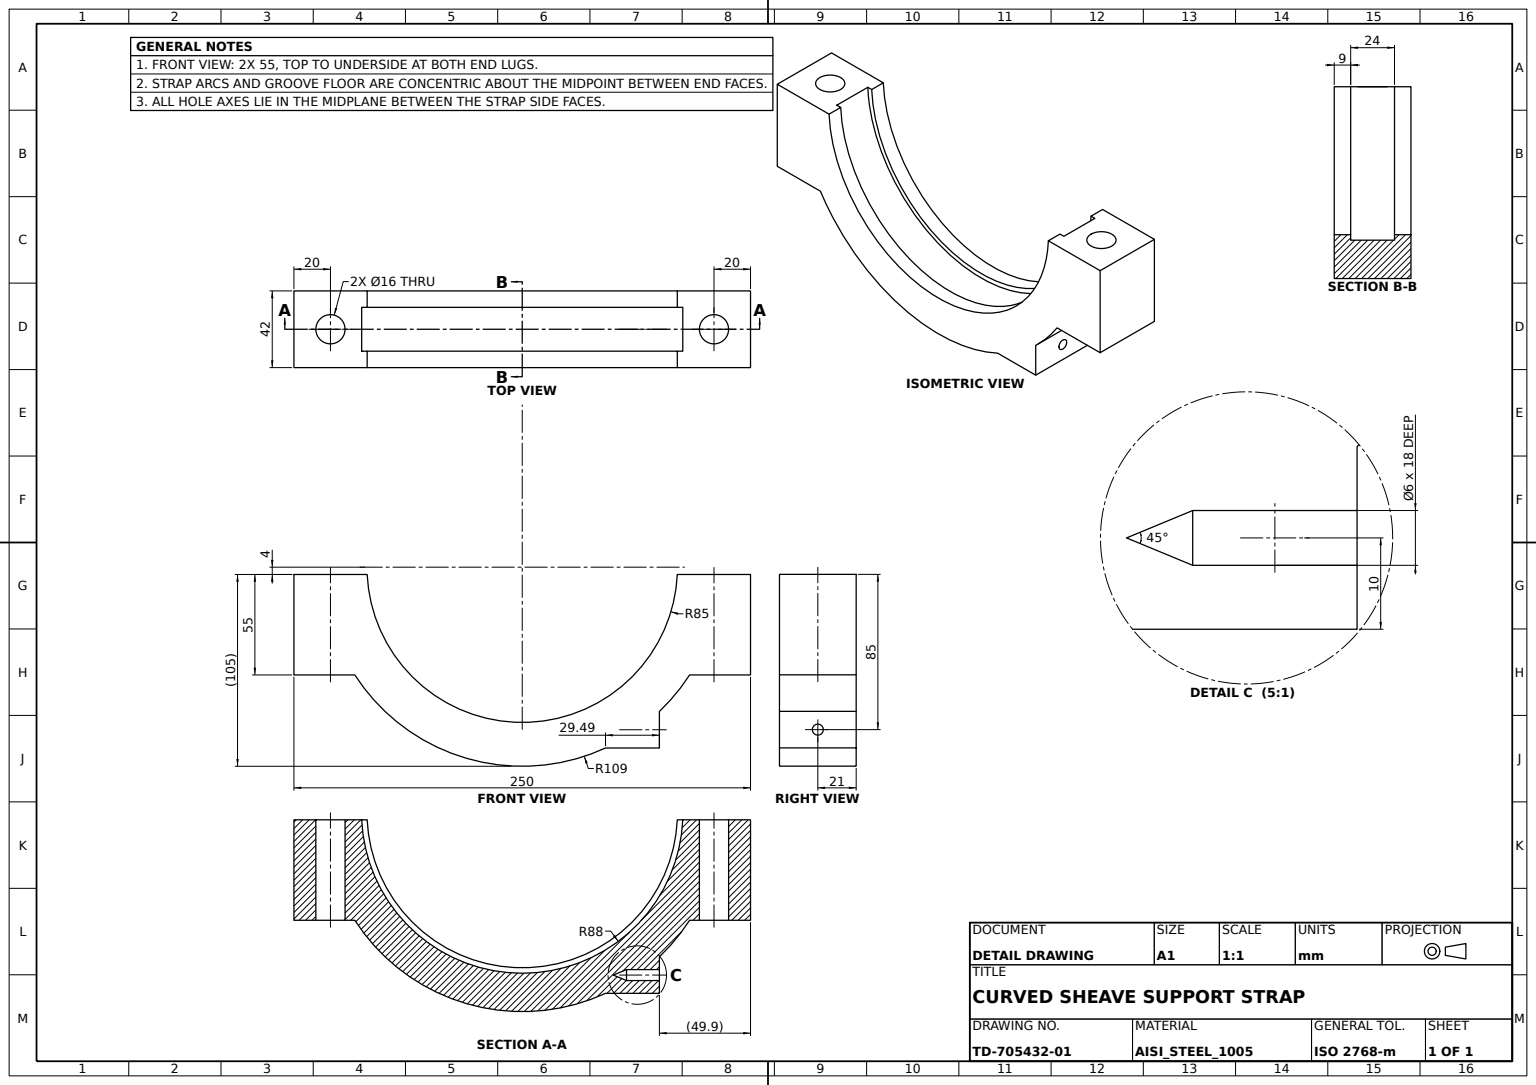
ISO-10303-21;
HEADER;
FILE_DESCRIPTION((''),'2;1');
FILE_NAME('','',(''),(''),'','','');
FILE_SCHEMA(('AUTOMOTIVE_DESIGN'));
ENDSEC;
DATA;
#1=APPLICATION_CONTEXT('');
#2=PRODUCT_CONTEXT('',#1,'mechanical');
#3=PRODUCT('','','',(#2));
#4=PRODUCT_DEFINITION_FORMATION('','',#3);
#5=PRODUCT_DEFINITION_CONTEXT('',#1,'design');
#6=PRODUCT_DEFINITION('','',#4,#5);
#7=PRODUCT_DEFINITION_SHAPE('','',#6);
#8=(LENGTH_UNIT()NAMED_UNIT(*)SI_UNIT(.MILLI.,.METRE.));
#9=(NAMED_UNIT(*)PLANE_ANGLE_UNIT()SI_UNIT($,.RADIAN.));
#10=(NAMED_UNIT(*)SI_UNIT($,.STERADIAN.)SOLID_ANGLE_UNIT());
#11=UNCERTAINTY_MEASURE_WITH_UNIT(LENGTH_MEASURE(0.005),#8,'distance_accuracy_value','');
#12=(GEOMETRIC_REPRESENTATION_CONTEXT(3)GLOBAL_UNCERTAINTY_ASSIGNED_CONTEXT((#11))GLOBAL_UNIT_ASSIGNED_CONTEXT((#8,#9,#10))REPRESENTATION_CONTEXT('',''));
#13=CARTESIAN_POINT('',(-55.,91.651514,21.));
#14=VERTEX_POINT('',#13);
#15=CARTESIAN_POINT('',(-55.,91.651514,-21.));
#16=VERTEX_POINT('',#15);
#17=DIRECTION('',(0.,0.,-1.));
#18=VECTOR('',#17,1000.);
#19=LINE('',#13,#18);
#20=EDGE_CURVE('',#14,#16,#19,.T.);
#21=ORIENTED_EDGE('',*,*,#20,.T.);
#22=CARTESIAN_POINT('',(-75.,75.099933,-21.));
#23=VERTEX_POINT('',#22);
#24=CARTESIAN_POINT('',(4.,0.,-21.));
#25=DIRECTION('',(0.,0.,1.));
#26=DIRECTION('',(0.,1.,0.));
#27=AXIS2_PLACEMENT_3D('',#24,#25,#26);
#28=CIRCLE('',#27,109.);
#29=EDGE_CURVE('',#16,#23,#28,.T.);
#30=ORIENTED_EDGE('',*,*,#29,.T.);
#31=CARTESIAN_POINT('',(-75.,75.099933,21.));
#32=VERTEX_POINT('',#31);
#33=LINE('',#31,#18);
#34=EDGE_CURVE('',#32,#23,#33,.T.);
#35=ORIENTED_EDGE('',*,*,#34,.F.);
#36=CARTESIAN_POINT('',(4.,0.,21.));
#37=AXIS2_PLACEMENT_3D('',#36,#25,#26);
#38=CIRCLE('',#37,109.);
#39=EDGE_CURVE('',#14,#32,#38,.T.);
#40=ORIENTED_EDGE('',*,*,#39,.F.);
#41=EDGE_LOOP('',(#21,#30,#35,#40));
#42=FACE_BOUND('',#41,.T.);
#43=DIRECTION('',(-1.,0.,0.));
#44=AXIS2_PLACEMENT_3D('',#36,#17,#43);
#45=CYLINDRICAL_SURFACE('',#44,109.);
#46=ADVANCED_FACE('',(#42),#45,.T.);
#47=CARTESIAN_POINT('',(0.,87.909044,12.));
#48=VERTEX_POINT('',#47);
#49=CARTESIAN_POINT('',(0.,87.909044,-12.));
#50=VERTEX_POINT('',#49);
#51=LINE('',#47,#18);
#52=EDGE_CURVE('',#48,#50,#51,.T.);
#53=ORIENTED_EDGE('',*,*,#52,.F.);
#54=CARTESIAN_POINT('',(0.,-87.909044,12.));
#55=VERTEX_POINT('',#54);
#56=CARTESIAN_POINT('',(4.,0.,12.));
#57=AXIS2_PLACEMENT_3D('',#56,#25,#26);
#58=CIRCLE('',#57,88.);
#59=EDGE_CURVE('',#55,#48,#58,.F.);
#60=ORIENTED_EDGE('',*,*,#59,.F.);
#61=CARTESIAN_POINT('',(0.,-87.909044,-12.));
#62=VERTEX_POINT('',#61);
#63=LINE('',#54,#18);
#64=EDGE_CURVE('',#55,#62,#63,.T.);
#65=ORIENTED_EDGE('',*,*,#64,.T.);
#66=CARTESIAN_POINT('',(4.,0.,-12.));
#67=AXIS2_PLACEMENT_3D('',#66,#25,#26);
#68=CIRCLE('',#67,88.);
#69=EDGE_CURVE('',#62,#50,#68,.F.);
#70=ORIENTED_EDGE('',*,*,#69,.T.);
#71=EDGE_LOOP('',(#53,#60,#65,#70));
#72=FACE_BOUND('',#71,.T.);
#73=AXIS2_PLACEMENT_3D('',#56,#17,#43);
#74=CYLINDRICAL_SURFACE('',#73,88.);
#75=ADVANCED_FACE('',(#72),#74,.F.);
#76=CARTESIAN_POINT('',(0.,-84.90583,-21.));
#77=VERTEX_POINT('',#76);
#78=CARTESIAN_POINT('',(0.,84.90583,-21.));
#79=VERTEX_POINT('',#78);
#80=AXIS2_PLACEMENT_3D('',#24,#17,#26);
#81=CIRCLE('',#80,85.);
#82=EDGE_CURVE('',#77,#79,#81,.T.);
#83=ORIENTED_EDGE('',*,*,#82,.T.);
#84=CARTESIAN_POINT('',(0.,84.90583,-12.));
#85=VERTEX_POINT('',#84);
#86=CARTESIAN_POINT('',(0.,84.90583,21.));
#87=LINE('',#86,#18);
#88=EDGE_CURVE('',#85,#79,#87,.T.);
#89=ORIENTED_EDGE('',*,*,#88,.F.);
#90=CARTESIAN_POINT('',(0.,-84.90583,-12.));
#91=VERTEX_POINT('',#90);
#92=AXIS2_PLACEMENT_3D('',#66,#17,#26);
#93=CIRCLE('',#92,85.);
#94=EDGE_CURVE('',#91,#85,#93,.T.);
#95=ORIENTED_EDGE('',*,*,#94,.F.);
#96=CARTESIAN_POINT('',(0.,-84.90583,21.));
#97=LINE('',#96,#18);
#98=EDGE_CURVE('',#91,#77,#97,.T.);
#99=ORIENTED_EDGE('',*,*,#98,.T.);
#100=EDGE_LOOP('',(#83,#89,#95,#99));
#101=FACE_BOUND('',#100,.T.);
#102=CYLINDRICAL_SURFACE('',#44,85.);
#103=ADVANCED_FACE('',(#101),#102,.F.);
#104=CARTESIAN_POINT('',(-55.,-97.,0.));
#105=VERTEX_POINT('',#104);
#106=CARTESIAN_POINT('',(-55.,-105.,0.));
#107=AXIS2_PLACEMENT_3D('',#106,#43,#26);
#108=CIRCLE('',#107,8.);
#109=EDGE_CURVE('',#105,#105,#108,.T.);
#110=ORIENTED_EDGE('',*,*,#109,.F.);
#111=EDGE_LOOP('',(#110));
#112=FACE_BOUND('',#111,.T.);
#113=CARTESIAN_POINT('',(-55.,-91.651514,21.));
#114=VERTEX_POINT('',#113);
#115=CARTESIAN_POINT('',(-55.,-125.,21.));
#116=VERTEX_POINT('',#115);
#117=DIRECTION('',(0.,-1.,0.));
#118=VECTOR('',#117,1000.);
#119=LINE('',#113,#118);
#120=EDGE_CURVE('',#114,#116,#119,.T.);
#121=ORIENTED_EDGE('',*,*,#120,.F.);
#122=CARTESIAN_POINT('',(-55.,-91.651514,-21.));
#123=VERTEX_POINT('',#122);
#124=LINE('',#113,#18);
#125=EDGE_CURVE('',#114,#123,#124,.T.);
#126=ORIENTED_EDGE('',*,*,#125,.T.);
#127=CARTESIAN_POINT('',(-55.,-125.,-21.));
#128=VERTEX_POINT('',#127);
#129=LINE('',#122,#118);
#130=EDGE_CURVE('',#123,#128,#129,.T.);
#131=ORIENTED_EDGE('',*,*,#130,.T.);
#132=LINE('',#115,#18);
#133=EDGE_CURVE('',#116,#128,#132,.T.);
#134=ORIENTED_EDGE('',*,*,#133,.F.);
#135=EDGE_LOOP('',(#121,#126,#131,#134));
#136=FACE_BOUND('',#135,.T.);
#137=DIRECTION('',(1.,0.,0.));
#138=AXIS2_PLACEMENT_3D('',#113,#137,#17);
#139=PLANE('',#138);
#140=ADVANCED_FACE('',(#112,#136),#139,.F.);
#141=CARTESIAN_POINT('',(0.,97.,0.));
#142=VERTEX_POINT('',#141);
#143=CARTESIAN_POINT('',(0.,105.,0.));
#144=AXIS2_PLACEMENT_3D('',#143,#43,#117);
#145=CIRCLE('',#144,8.);
#146=EDGE_CURVE('',#142,#142,#145,.T.);
#147=ORIENTED_EDGE('',*,*,#146,.F.);
#148=EDGE_LOOP('',(#147));
#149=FACE_BOUND('',#148,.T.);
#150=CARTESIAN_POINT('',(-55.,97.,0.));
#151=VERTEX_POINT('',#150);
#152=CARTESIAN_POINT('',(-55.,105.,0.));
#153=AXIS2_PLACEMENT_3D('',#152,#137,#117);
#154=CIRCLE('',#153,8.);
#155=EDGE_CURVE('',#151,#151,#154,.T.);
#156=ORIENTED_EDGE('',*,*,#155,.F.);
#157=EDGE_LOOP('',(#156));
#158=FACE_BOUND('',#157,.T.);
#159=CARTESIAN_POINT('',(5.5,105.,0.));
#160=AXIS2_PLACEMENT_3D('',#159,#43,#25);
#161=CYLINDRICAL_SURFACE('',#160,8.);
#162=ADVANCED_FACE('',(#149,#158),#161,.F.);
#163=CARTESIAN_POINT('',(-95.,45.607017,-21.));
#164=VERTEX_POINT('',#163);
#165=EDGE_CURVE('',#164,#123,#28,.T.);
#166=ORIENTED_EDGE('',*,*,#165,.T.);
#167=ORIENTED_EDGE('',*,*,#125,.F.);
#168=CARTESIAN_POINT('',(-95.,45.607017,21.));
#169=VERTEX_POINT('',#168);
#170=EDGE_CURVE('',#169,#114,#38,.T.);
#171=ORIENTED_EDGE('',*,*,#170,.F.);
#172=LINE('',#168,#18);
#173=EDGE_CURVE('',#169,#164,#172,.T.);
#174=ORIENTED_EDGE('',*,*,#173,.T.);
#175=EDGE_LOOP('',(#166,#167,#171,#174));
#176=FACE_BOUND('',#175,.T.);
#177=ADVANCED_FACE('',(#176),#45,.T.);
#178=ORIENTED_EDGE('',*,*,#130,.F.);
#179=ORIENTED_EDGE('',*,*,#165,.F.);
#180=CARTESIAN_POINT('',(-95.,75.099933,-21.));
#181=VERTEX_POINT('',#180);
#182=LINE('',#180,#118);
#183=EDGE_CURVE('',#181,#164,#182,.T.);
#184=ORIENTED_EDGE('',*,*,#183,.F.);
#185=VECTOR('',#43,1000.);
#186=LINE('',#22,#185);
#187=EDGE_CURVE('',#23,#181,#186,.T.);
#188=ORIENTED_EDGE('',*,*,#187,.F.);
#189=ORIENTED_EDGE('',*,*,#29,.F.);
#190=CARTESIAN_POINT('',(-55.,125.,-21.));
#191=VERTEX_POINT('',#190);
#192=LINE('',#190,#118);
#193=EDGE_CURVE('',#191,#16,#192,.T.);
#194=ORIENTED_EDGE('',*,*,#193,.F.);
#195=CARTESIAN_POINT('',(0.,125.,-21.));
#196=VERTEX_POINT('',#195);
#197=LINE('',#195,#185);
#198=EDGE_CURVE('',#196,#191,#197,.T.);
#199=ORIENTED_EDGE('',*,*,#198,.F.);
#200=VECTOR('',#26,1000.);
#201=LINE('',#78,#200);
#202=EDGE_CURVE('',#79,#196,#201,.T.);
#203=ORIENTED_EDGE('',*,*,#202,.F.);
#204=ORIENTED_EDGE('',*,*,#82,.F.);
#205=CARTESIAN_POINT('',(0.,-125.,-21.));
#206=VERTEX_POINT('',#205);
#207=LINE('',#205,#200);
#208=EDGE_CURVE('',#206,#77,#207,.T.);
#209=ORIENTED_EDGE('',*,*,#208,.F.);
#210=VECTOR('',#137,1000.);
#211=LINE('',#127,#210);
#212=EDGE_CURVE('',#128,#206,#211,.T.);
#213=ORIENTED_EDGE('',*,*,#212,.F.);
#214=EDGE_LOOP('',(#178,#179,#184,#188,#189,#194,#199,#203,#204,#209,#213));
#215=FACE_BOUND('',#214,.T.);
#216=AXIS2_PLACEMENT_3D('',#24,#25,#137);
#217=PLANE('',#216);
#218=ADVANCED_FACE('',(#215),#217,.F.);
#219=CARTESIAN_POINT('',(-95.,75.099933,21.));
#220=VERTEX_POINT('',#219);
#221=LINE('',#219,#118);
#222=EDGE_CURVE('',#220,#169,#221,.T.);
#223=ORIENTED_EDGE('',*,*,#222,.T.);
#224=ORIENTED_EDGE('',*,*,#170,.T.);
#225=ORIENTED_EDGE('',*,*,#120,.T.);
#226=CARTESIAN_POINT('',(0.,-125.,21.));
#227=VERTEX_POINT('',#226);
#228=LINE('',#115,#210);
#229=EDGE_CURVE('',#116,#227,#228,.T.);
#230=ORIENTED_EDGE('',*,*,#229,.T.);
#231=VERTEX_POINT('',#96);
#232=LINE('',#226,#200);
#233=EDGE_CURVE('',#227,#231,#232,.T.);
#234=ORIENTED_EDGE('',*,*,#233,.T.);
#235=VERTEX_POINT('',#86);
#236=AXIS2_PLACEMENT_3D('',#36,#17,#26);
#237=CIRCLE('',#236,85.);
#238=EDGE_CURVE('',#231,#235,#237,.T.);
#239=ORIENTED_EDGE('',*,*,#238,.T.);
#240=CARTESIAN_POINT('',(0.,125.,21.));
#241=VERTEX_POINT('',#240);
#242=LINE('',#86,#200);
#243=EDGE_CURVE('',#235,#241,#242,.T.);
#244=ORIENTED_EDGE('',*,*,#243,.T.);
#245=CARTESIAN_POINT('',(-55.,125.,21.));
#246=VERTEX_POINT('',#245);
#247=LINE('',#240,#185);
#248=EDGE_CURVE('',#241,#246,#247,.T.);
#249=ORIENTED_EDGE('',*,*,#248,.T.);
#250=LINE('',#245,#118);
#251=EDGE_CURVE('',#246,#14,#250,.T.);
#252=ORIENTED_EDGE('',*,*,#251,.T.);
#253=ORIENTED_EDGE('',*,*,#39,.T.);
#254=LINE('',#31,#185);
#255=EDGE_CURVE('',#32,#220,#254,.T.);
#256=ORIENTED_EDGE('',*,*,#255,.T.);
#257=EDGE_LOOP('',(#223,#224,#225,#230,#234,#239,#244,#249,#252,#253,#256));
#258=FACE_BOUND('',#257,.T.);
#259=AXIS2_PLACEMENT_3D('',#36,#25,#137);
#260=PLANE('',#259);
#261=ADVANCED_FACE('',(#258),#260,.T.);
#262=CARTESIAN_POINT('',(0.,-84.90583,12.));
#263=VERTEX_POINT('',#262);
#264=CARTESIAN_POINT('',(0.,84.90583,12.));
#265=VERTEX_POINT('',#264);
#266=AXIS2_PLACEMENT_3D('',#56,#17,#26);
#267=CIRCLE('',#266,85.);
#268=EDGE_CURVE('',#263,#265,#267,.T.);
#269=ORIENTED_EDGE('',*,*,#268,.F.);
#270=LINE('',#54,#200);
#271=EDGE_CURVE('',#55,#263,#270,.T.);
#272=ORIENTED_EDGE('',*,*,#271,.F.);
#273=ORIENTED_EDGE('',*,*,#59,.T.);
#274=LINE('',#264,#200);
#275=EDGE_CURVE('',#265,#48,#274,.T.);
#276=ORIENTED_EDGE('',*,*,#275,.F.);
#277=EDGE_LOOP('',(#269,#272,#273,#276));
#278=FACE_BOUND('',#277,.T.);
#279=PLANE('',#73);
#280=ADVANCED_FACE('',(#278),#279,.T.);
#281=CARTESIAN_POINT('',(-85.,75.099933,-3.));
#282=VERTEX_POINT('',#281);
#283=CARTESIAN_POINT('',(-85.,75.099933,0.));
#284=AXIS2_PLACEMENT_3D('',#283,#117,#17);
#285=CIRCLE('',#284,3.);
#286=EDGE_CURVE('',#282,#282,#285,.T.);
#287=ORIENTED_EDGE('',*,*,#286,.T.);
#288=EDGE_LOOP('',(#287));
#289=FACE_BOUND('',#288,.T.);
#290=LINE('',#219,#18);
#291=EDGE_CURVE('',#220,#181,#290,.T.);
#292=ORIENTED_EDGE('',*,*,#291,.F.);
#293=ORIENTED_EDGE('',*,*,#255,.F.);
#294=ORIENTED_EDGE('',*,*,#34,.T.);
#295=ORIENTED_EDGE('',*,*,#187,.T.);
#296=EDGE_LOOP('',(#292,#293,#294,#295));
#297=FACE_BOUND('',#296,.T.);
#298=AXIS2_PLACEMENT_3D('',#31,#117,#17);
#299=PLANE('',#298);
#300=ADVANCED_FACE('',(#289,#297),#299,.F.);
#301=ORIENTED_EDGE('',*,*,#109,.T.);
#302=EDGE_LOOP('',(#301));
#303=FACE_BOUND('',#302,.T.);
#304=CARTESIAN_POINT('',(0.,-105.,8.));
#305=VERTEX_POINT('',#304);
#306=CARTESIAN_POINT('',(0.,-105.,0.));
#307=AXIS2_PLACEMENT_3D('',#306,#43,#25);
#308=CIRCLE('',#307,8.);
#309=EDGE_CURVE('',#305,#305,#308,.F.);
#310=ORIENTED_EDGE('',*,*,#309,.T.);
#311=EDGE_LOOP('',(#310));
#312=FACE_BOUND('',#311,.T.);
#313=CARTESIAN_POINT('',(5.5,-105.,0.));
#314=AXIS2_PLACEMENT_3D('',#313,#43,#25);
#315=CYLINDRICAL_SURFACE('',#314,8.);
#316=ADVANCED_FACE('',(#303,#312),#315,.F.);
#317=CARTESIAN_POINT('',(-85.,57.099933,-3.));
#318=VERTEX_POINT('',#317);
#319=CARTESIAN_POINT('',(-85.,57.099933,0.));
#320=AXIS2_PLACEMENT_3D('',#319,#117,#17);
#321=CIRCLE('',#320,3.);
#322=EDGE_CURVE('',#318,#318,#321,.F.);
#323=ORIENTED_EDGE('',*,*,#322,.F.);
#324=EDGE_LOOP('',(#323));
#325=FACE_BOUND('',#324,.T.);
#326=ORIENTED_EDGE('',*,*,#286,.F.);
#327=EDGE_LOOP('',(#326));
#328=FACE_BOUND('',#327,.T.);
#329=CYLINDRICAL_SURFACE('',#284,3.);
#330=ADVANCED_FACE('',(#325,#328),#329,.F.);
#331=ORIENTED_EDGE('',*,*,#248,.F.);
#332=LINE('',#240,#18);
#333=EDGE_CURVE('',#241,#196,#332,.T.);
#334=ORIENTED_EDGE('',*,*,#333,.T.);
#335=ORIENTED_EDGE('',*,*,#198,.T.);
#336=LINE('',#245,#18);
#337=EDGE_CURVE('',#246,#191,#336,.T.);
#338=ORIENTED_EDGE('',*,*,#337,.F.);
#339=EDGE_LOOP('',(#331,#334,#335,#338));
#340=FACE_BOUND('',#339,.T.);
#341=AXIS2_PLACEMENT_3D('',#240,#117,#17);
#342=PLANE('',#341);
#343=ADVANCED_FACE('',(#340),#342,.F.);
#344=ORIENTED_EDGE('',*,*,#243,.F.);
#345=EDGE_CURVE('',#235,#265,#87,.T.);
#346=ORIENTED_EDGE('',*,*,#345,.T.);
#347=ORIENTED_EDGE('',*,*,#275,.T.);
#348=ORIENTED_EDGE('',*,*,#52,.T.);
#349=LINE('',#84,#200);
#350=EDGE_CURVE('',#85,#50,#349,.T.);
#351=ORIENTED_EDGE('',*,*,#350,.F.);
#352=ORIENTED_EDGE('',*,*,#88,.T.);
#353=ORIENTED_EDGE('',*,*,#202,.T.);
#354=ORIENTED_EDGE('',*,*,#333,.F.);
#355=EDGE_LOOP('',(#344,#346,#347,#348,#351,#352,#353,#354));
#356=FACE_BOUND('',#355,.T.);
#357=ORIENTED_EDGE('',*,*,#146,.T.);
#358=EDGE_LOOP('',(#357));
#359=FACE_BOUND('',#358,.T.);
#360=AXIS2_PLACEMENT_3D('',#86,#43,#117);
#361=PLANE('',#360);
#362=ADVANCED_FACE('',(#356,#359),#361,.F.);
#363=ORIENTED_EDGE('',*,*,#309,.F.);
#364=EDGE_LOOP('',(#363));
#365=FACE_BOUND('',#364,.T.);
#366=ORIENTED_EDGE('',*,*,#233,.F.);
#367=LINE('',#226,#18);
#368=EDGE_CURVE('',#227,#206,#367,.T.);
#369=ORIENTED_EDGE('',*,*,#368,.T.);
#370=ORIENTED_EDGE('',*,*,#208,.T.);
#371=ORIENTED_EDGE('',*,*,#98,.F.);
#372=LINE('',#61,#200);
#373=EDGE_CURVE('',#62,#91,#372,.T.);
#374=ORIENTED_EDGE('',*,*,#373,.F.);
#375=ORIENTED_EDGE('',*,*,#64,.F.);
#376=ORIENTED_EDGE('',*,*,#271,.T.);
#377=EDGE_CURVE('',#231,#263,#97,.T.);
#378=ORIENTED_EDGE('',*,*,#377,.F.);
#379=EDGE_LOOP('',(#366,#369,#370,#371,#374,#375,#376,#378));
#380=FACE_BOUND('',#379,.T.);
#381=AXIS2_PLACEMENT_3D('',#226,#43,#25);
#382=PLANE('',#381);
#383=ADVANCED_FACE('',(#365,#380),#382,.F.);
#384=ORIENTED_EDGE('',*,*,#291,.T.);
#385=ORIENTED_EDGE('',*,*,#183,.T.);
#386=ORIENTED_EDGE('',*,*,#173,.F.);
#387=ORIENTED_EDGE('',*,*,#222,.F.);
#388=EDGE_LOOP('',(#384,#385,#386,#387));
#389=FACE_BOUND('',#388,.T.);
#390=AXIS2_PLACEMENT_3D('',#219,#137,#26);
#391=PLANE('',#390);
#392=ADVANCED_FACE('',(#389),#391,.F.);
#393=ORIENTED_EDGE('',*,*,#322,.T.);
#394=EDGE_LOOP('',(#393));
#395=FACE_BOUND('',#394,.T.);
#396=CARTESIAN_POINT('',(-85.,49.857293,0.));
#397=VERTEX_POINT('',#396);
#398=VERTEX_LOOP('',#397);
#399=FACE_BOUND('',#398,.T.);
#400=AXIS2_PLACEMENT_3D('',#319,#26,#25);
#401=CONICAL_SURFACE('',#400,3.,0.392699082);
#402=ADVANCED_FACE('',(#395,#399),#401,.F.);
#403=ORIENTED_EDGE('',*,*,#350,.T.);
#404=ORIENTED_EDGE('',*,*,#69,.F.);
#405=ORIENTED_EDGE('',*,*,#373,.T.);
#406=ORIENTED_EDGE('',*,*,#94,.T.);
#407=EDGE_LOOP('',(#403,#404,#405,#406));
#408=FACE_BOUND('',#407,.T.);
#409=AXIS2_PLACEMENT_3D('',#66,#17,#43);
#410=PLANE('',#409);
#411=ADVANCED_FACE('',(#408),#410,.F.);
#412=ORIENTED_EDGE('',*,*,#155,.T.);
#413=EDGE_LOOP('',(#412));
#414=FACE_BOUND('',#413,.T.);
#415=ORIENTED_EDGE('',*,*,#193,.T.);
#416=ORIENTED_EDGE('',*,*,#20,.F.);
#417=ORIENTED_EDGE('',*,*,#251,.F.);
#418=ORIENTED_EDGE('',*,*,#337,.T.);
#419=EDGE_LOOP('',(#415,#416,#417,#418));
#420=FACE_BOUND('',#419,.T.);
#421=AXIS2_PLACEMENT_3D('',#245,#137,#17);
#422=PLANE('',#421);
#423=ADVANCED_FACE('',(#414,#420),#422,.F.);
#424=ORIENTED_EDGE('',*,*,#377,.T.);
#425=ORIENTED_EDGE('',*,*,#268,.T.);
#426=ORIENTED_EDGE('',*,*,#345,.F.);
#427=ORIENTED_EDGE('',*,*,#238,.F.);
#428=EDGE_LOOP('',(#424,#425,#426,#427));
#429=FACE_BOUND('',#428,.T.);
#430=ADVANCED_FACE('',(#429),#102,.F.);
#431=ORIENTED_EDGE('',*,*,#212,.T.);
#432=ORIENTED_EDGE('',*,*,#368,.F.);
#433=ORIENTED_EDGE('',*,*,#229,.F.);
#434=ORIENTED_EDGE('',*,*,#133,.T.);
#435=EDGE_LOOP('',(#431,#432,#433,#434));
#436=FACE_BOUND('',#435,.T.);
#437=AXIS2_PLACEMENT_3D('',#115,#26,#25);
#438=PLANE('',#437);
#439=ADVANCED_FACE('',(#436),#438,.F.);
#440=CLOSED_SHELL('',(#46,#75,#103,#140,#162,#177,#218,#261,#280,#300,#316,#330,#343,#362,#383,#392,#402,#411,#423,#430,#439));
#441=MANIFOLD_SOLID_BREP('',#440);
#442=ADVANCED_BREP_SHAPE_REPRESENTATION('',(#441),#12);
#443=SHAPE_DEFINITION_REPRESENTATION(#7,#442);
ENDSEC;
END-ISO-10303-21;
